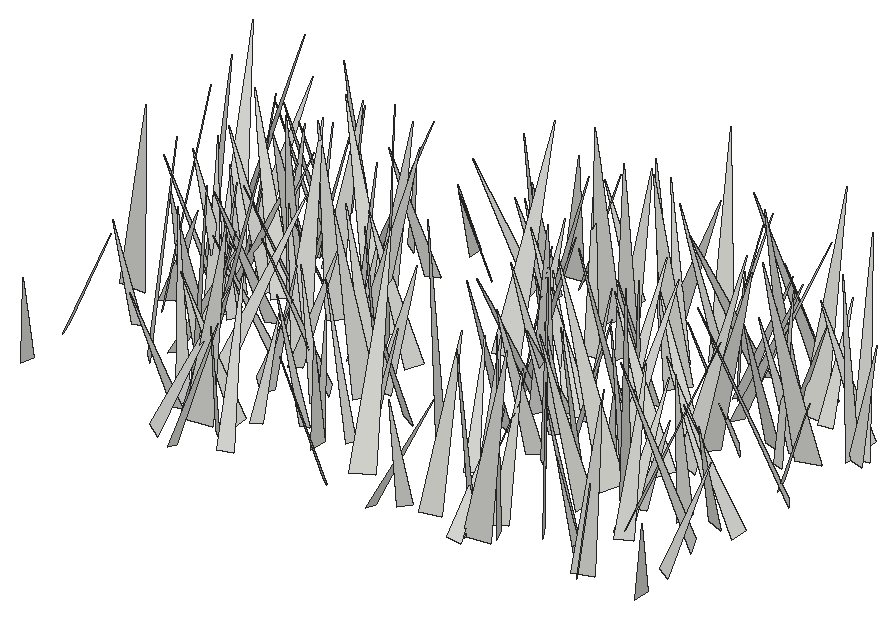
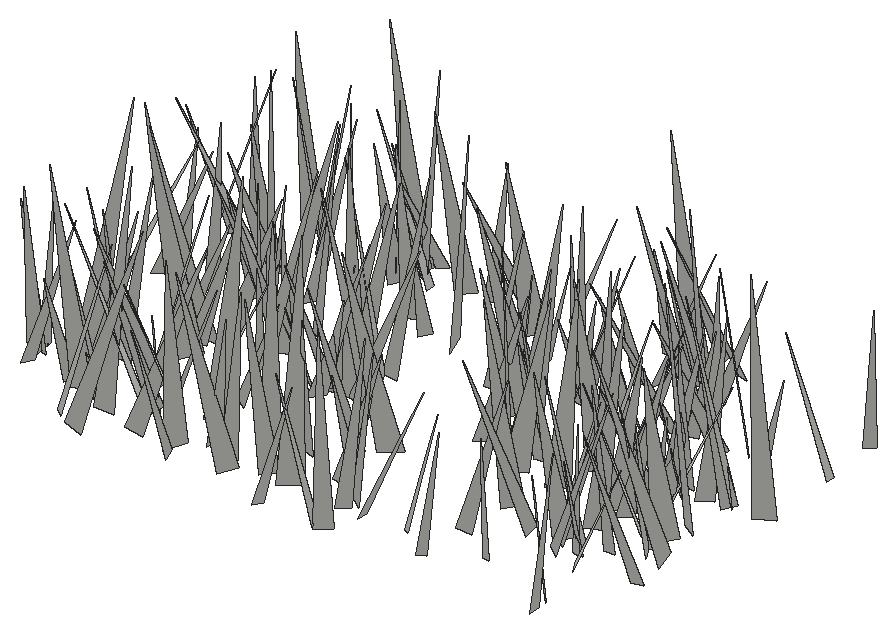
# SketchUp Ruby script. Lengths in inches.
U = 1.inch
M = Sketchup.active_model
def pt(a) = Geom::Point3d.new(a.map { |v| v * U })
def face(e, loops, mat)
  f = e.add_face(loops[0].map { |a| pt(a) })
  loops[1..].each { |l| e.add_face(l.map { |a| pt(a) }).erase! }
  f.material = f.back_material = mat if mat
  f
end
# faces: each face lists its corners as indices into pts; further lists are holes
def faces(e, pts, list, mat = nil) = list.each { |f| face(e, (f[0].is_a?(Array) ? f : [f]).map { |l| l.map { |i| pts[i] } }, mat) }
# xy, xz, yz: faces in a plane at the given z, y or x. An outline is a flat list of corners, or four numbers for a rectangle; further outlines are holes
def ring(l) = l.size == 4 ? [[l[0], l[1]], [l[2], l[1]], [l[2], l[3]], [l[0], l[3]]] : l.each_slice(2).to_a
def flat(e, list, mat, &to3) = list.each { |f| face(e, (f[0].is_a?(Array) ? f : [f]).map { |l| ring(l).map { |u, v| to3.(u, v) } }, mat) }
def xy(e, z, list, mat = nil) = flat(e, list, mat) { |x, y| [x, y, z] }
def xz(e, y, list, mat = nil) = flat(e, list, mat) { |x, z| [x, y, z] }
def yz(e, x, list, mat = nil) = flat(e, list, mat) { |y, z| [x, y, z] }
def lines(e, pts, list) = list.each { |a, b| e.add_line(pt(pts[a]), pt(pts[b])) }
# prism: a flat outline (further loops are holes) pulled along v
def prism(e, loops, v, mat = nil)
  f = face(e, loops, mat); d = Geom::Vector3d.new(v.map { |x| x * U })
  f.pushpull(f.normal.samedirection?(d) ? d.length : -d.length)
end
def box(e, o, s, mat = nil) = prism(e, [[o, [o[0] + s[0], o[1], o[2]], [o[0] + s[0], o[1] + s[1], o[2]], [o[0], o[1] + s[1], o[2]]]], [0, 0, s[2]], mat)
def at(x, y, z, deg = 0) = Geom::Transformation.translation(pt([x, y, z])) * Geom::Transformation.rotation(ORIGIN, Z_AXIS, deg.degrees)
def axes(o, x, y, z) = Geom::Transformation.new([*x, 0, *y, 0, *z, 0, *pt(o).to_a, 1])
def part(name) = M.definitions.add(name)
# library, detail: a bought-in or finely detailed component or shape, given as its bounding box
def library(name, o, s) = part(name).tap { |d| box(d.entities, o, s) }
def detail(e, o, s) = box(e.add_group.entities, o, s)
def put(e, d, t, mat = nil) = e.add_instance(d, t).tap { |i| i.material = mat if mat }
def group(e, t, mat = nil) = e.add_group.tap { |g| g.transformation = t; g.material = mat if mat }.entities
root = M.entities
c1 = part("fur_instance\#9")
p = [[0.8125,0,1.79],[0.67,-0.02,1.48],[0,-0.11,0],[0,0.11,0]]
faces(c1.entities,p,[[0,1,2,3]])
put(root,c1,axes([515.02,377.61,-21.66],[4.28943,0.41298,0.87796],[0.18379,-4.25331,1.1028],[-0.95267,1.03894,4.16576]))
put(root,c1,axes([501.53,380.35,-21.66],[3.7269,-2.05729,0.24824],[-1.97365,-3.67974,-0.86491],[-0.63149,-0.64103,4.16823]))
put(root,c1,axes([536.71,380.03,-21.66],[-1.94061,6.26278,4.61542],[7.19839,3.24975,-1.38302],[2.95087,-3.80883,6.40903]))
put(root,c1,axes([548.84,380.86,-21.66],[3.9114,-1.46291,0.01114],[-1.40736,-3.77134,-1.11157],[-0.39945,-1.03737,4.02536]))
put(root,c1,axes([516.36,380.32,-21.66],[2.79226,2.81825,2.22878],[3.51982,-2.71249,-0.9798],[-0.72174,-2.32521,3.84438]))
put(root,c1,axes([525.09,379.86,-21.66],[-2.96371,-3.18096,0.56073],[-3.21747,2.84043,-0.89238],[-0.28422,1.01488,4.25508]))
put(root,c1,axes([530.68,380.6,-21.66],[2.96444,-3.24193,0.90441],[-3.19075,-3.09049,-0.61962],[-1.07107,0.23387,4.34903]))
put(root,c1,axes([512.91,378.43,-21.66],[2.64419,5.03318,0.33977],[4.95036,-2.51506,-1.26831],[0.97076,-0.88412,5.54221]))
put(root,c1,axes([514.43,380.82,-21.66],[3.42079,-7.2545,1.9343],[-7.49487,-3.17419,1.34998],[0.44283,2.31686,7.90614]))
put(root,c1,axes([535.65,381,-21.66],[3.71105,4.69804,3.51461],[5.68502,-3.90755,-0.77947],[-1.45074,-3.29476,5.93598]))
put(root,c1,axes([529.1,379.28,-21.66],[4.45979,0.0367,0.09292],[0.01604,-4.35825,0.95137],[-0.0986,0.95079,4.35729]))
put(root,c1,axes([544.46,380.66,-21.66],[3.53738,-5.32848,1.99163],[-5.66565,-3.51029,0.67133],[-0.50966,2.039,6.36044]))
put(root,c1,axes([512.27,381.46,-21.66],[-0.63614,-4.28295,0.71253],[-4.25699,0.4736,-0.95381],[-0.85404,0.8295,4.22357]))
put(root,c1,axes([536.11,380.16,-21.66],[4.52049,-0.19473,1.20973],[-0.39564,-4.60837,0.73662],[-1.15967,0.81315,4.46432]))
put(root,c1,axes([535.64,379.1,-21.66],[-1.08496,4.24211,0.2137],[4.12597,1.10497,-0.98676],[1.00871,0.04308,4.26602]))
put(root,c1,axes([517.94,379.03,-21.66],[-0.8094,5.47668,0.09308],[5.43232,0.79056,0.72297],[-0.70181,-0.19701,5.48875]))
put(root,c1,axes([534.66,381.58,-21.66],[5.44749,2.02001,0.26599],[2.02291,-5.27178,-1.39377],[0.24298,-1.39796,5.64031]))
put(root,c1,axes([542.72,382.29,-21.66],[3.69815,0.46024,1.83595],[1.02421,-3.87534,-1.09159],[-1.5917,-1.42435,3.56322]))
put(root,c1,axes([532.54,380.76,-21.66],[-2.8521,5.31504,2.52319],[5.50682,3.39878,-0.93481],[2.07151,-1.71732,5.95905]))
put(root,c1,axes([542.52,382.71,-21.66],[-4.88015,-2.78524,1.52655],[-2.68194,5.11285,0.7548],[1.7015,0.07051,5.5681]))
put(root,c1,axes([544.2,380.46,-21.66],[4.62309,3.63215,1.82021],[3.50208,-4.96051,1.00367],[-2.05939,-0.28182,5.79293]))
put(root,c1,axes([516.47,382.34,-21.66],[-5.33847,-0.05884,0.40473],[-0.0096,5.31499,0.64603],[0.40887,-0.64342,5.29956]))
put(root,c1,axes([521.91,383.08,-21.66],[4.60045,-1.39498,0.802],[-1.20201,-4.59424,-1.0961],[-1.06973,-0.83684,4.68067]))
put(root,c1,axes([537.4,381.3125,-21.66],[-5.47988,-2.79163,2.54101],[-3.31815,5.69792,-0.89593],[1.79996,2.00489,6.08438]))
put(root,c1,axes([539.3,383.32,-21.66],[4.52719,2.71843,2.25301],[3.1828,-4.72799,-0.69084],[-1.52829,-1.79378,5.23527]))
put(root,c1,axes([513,382.04,-21.66],[-6.34859,-2.07949,3.15929],[-2.7531,6.77324,-1.07409],[2.59343,2.09974,6.59357]))
put(root,c1,axes([512.7,381.8,-21.66],[5.61181,2.09612,1.30854],[1.89864,-5.73587,1.04566],[-1.58152,0.55181,5.89854]))
put(root,c1,axes([536.69,382.27,-21.66],[3.58302,-2.92408,2.58959],[-3.63927,-3.77537,0.77237],[-1.41842,2.30013,4.5598]))
put(root,c1,axes([514.33,381.36,-21.66],[2.31766,5.02687,0.82298],[4.84651,-2.45447,1.34356],[-1.56781,-0.15629,5.3699]))
put(root,c1,axes([512.23,382.14,-21.66],[-5.96382,1.04535,0.88629],[0.82737,5.90096,-1.39268],[1.09259,1.23747,5.8924]))
put(root,c1,axes([517.27,382.95,-21.66],[-2.50227,2.59124,1.1484],[2.47228,2.74461,-0.80603],[1.38608,-0.21748,3.51087]))
put(root,c1,axes([521,384.45,-21.66],[-1.15878,-4.12917,1.68532],[-4.31214,1.48176,0.66553],[1.13832,1.40977,4.23673]))
put(root,c1,axes([548.17,383.84,-21.66],[1.81296,4.05322,0.9149],[4.0683,-1.5284,-1.29051],[0.84535,-1.3371,4.24853]))
put(root,c1,axes([519.85,384.42,-21.66],[-1.05409,-4.02831,1.60299],[-4.27873,0.70037,-1.05356],[-0.69957,1.78611,4.02845]))
put(root,c1,axes([526.15,382.11,-21.66],[-5.32969,5.59283,1.04722],[5.46672,5.43108,-1.18331],[1.57839,0.07463,7.63447]))
put(root,c1,axes([500.93,384.9,-21.66],[4.64757,1.11707,0.03174],[1.0994,-4.54603,-0.98676],[0.20042,-0.96672,4.67697]))
put(root,c1,axes([533.22,385.27,-21.66],[1.79677,-5.19077,1.98742],[-5.55817,-1.66844,0.66734],[0.02536,2.09632,5.45226]))
put(root,c1,axes([512.23,383.71,-21.66],[7.1658,2.76652,1.69463],[2.58302,-7.35112,1.0785],[-1.96302,0.42601,7.60521]))
put(root,c1,axes([510.76,386.04,-21.66],[1.65267,-3.08975,1.39314],[-3.11179,-1.99748,-0.7386],[-1.34319,0.82596,3.42525]))
put(root,c1,axes([523.22,384.66,-21.66],[-5.0928,-0.09663,0.30052],[-0.16718,4.94609,-1.24277],[0.26777,1.25023,4.93978]))
put(root,c1,axes([547.4375,387.625,-21.66],[-6.20771,-3.16783,0.82777],[-3.08728,6.25411,0.78157],[1.09042,-0.32718,6.92531]))
put(root,c1,axes([524.13,385.21,-21.66],[3.78689,-0.0231,1.24793],[-0.32688,-3.86581,0.92039],[-1.20458,0.97644,3.67342]))
put(root,c1,axes([539.24,387.36,-21.66],[-6.05597,0.77226,2.0179],[1.21073,6.18666,1.26588],[1.78953,-1.57224,5.97233]))
put(root,c1,axes([507.14,385.13,-21.66],[4.85297,5.01471,2.08252],[4.89411,-5.24941,1.23566],[-2.35199,-0.5761,6.86817]))
put(root,c1,axes([529.1,386.17,-21.66],[-7.32615,-2.19993,2.60741],[-2.57876,7.61493,-0.82074],[2.23345,1.57604,7.60517]))
put(root,c1,axes([543.68,385.6,-21.66],[3.74309,-3.05687,3.19875],[-4.02453,-4.09315,0.7978],[-1.83838,2.73658,4.76642]))
put(root,c1,axes([514.06,387.06,-21.66],[2.61371,2.45973,0.53308],[2.49517,-2.43181,-1.01309],[0.32949,-1.09634,3.44317]))
put(root,c1,axes([524.23,388.98,-21.66],[-1.58112,-4.73276,0.31075],[-4.65779,1.61119,0.83937],[0.89473,0.02406,4.91878]))
put(root,c1,axes([515.36,386.55,-21.66],[4.20313,-0.16718,1.34956],[-0.39887,-4.34286,0.70427],[-1.30006,0.79192,4.14708]))
put(root,c1,axes([518.23,388.9,-21.66],[-5.1626,-2.88411,0.4563],[-2.82641,5.16852,0.6903],[0.7333,-0.3834,5.87316]))
put(root,c1,axes([507.92,386.7,-21.66],[4.70172,-1.10111,0.26171],[-1.12934,-4.49092,1.39405],[0.07438,1.41645,4.62334]))
put(root,c1,axes([503.99,387.99,-21.66],[-0.09942,-3.58739,1.13729],[-3.70553,-0.10534,-0.65623],[-0.65715,1.13676,3.52826]))
put(root,c1,axes([518.55,387.15,-21.66],[-0.54656,4.2534,1.19948],[4.32093,0.26075,1.04426],[-0.92722,-1.29209,4.15928]))
put(root,c1,axes([531.24,386.32,-21.66],[-2.96108,3.10315,0.36366],[3.04624,2.97875,-0.6142],[0.69442,0.16515,4.24503]))
put(root,c1,axes([543.19,386.12,-21.66],[-2.46279,4.53865,0.90199],[4.34757,2.61941,-1.3098],[1.58479,-0.13272,4.99491]))
put(root,c1,axes([520.41,389.55,-21.66],[4.49335,-4.83843,2.48866],[-4.8443,-5.0271,-1.02712],[-2.47721,1.05444,6.5227]))
put(root,c1,axes([511.64,386.47,-21.66],[1.69788,6.23349,0.03172],[6.16311,-1.67374,-0.97718],[0.93461,-0.28707,6.38626]))
put(root,c1,axes([546.875,390.42,-21.66],[-0.66532,-4.77379,0.4836],[-4.67341,0.75535,1.0268],[1.0873,0.32553,4.70929]))
put(root,c1,axes([542.84,387.09,-21.66],[6.48449,2.8801,0.19854],[2.8437,-6.45643,0.78158],[-0.49773,0.63448,7.05214]))
put(root,c1,axes([536.36,390.45,-21.66],[-2.50316,-5.2047,1.47138],[-5.2002,2.76171,0.92225],[1.48721,0.89649,5.70124]))
put(root,c1,axes([532.87,390.5,-21.66],[1.51569,-5.39227,1.25729],[-5.41404,-1.71643,-0.83467],[-1.15995,0.96539,5.5387]))
put(root,c1,axes([544.9375,389.91,-21.66],[-4.81176,0.83188,2.6308],[1.27412,5.3609,0.63523],[2.44739,-1.15538,4.84165]))
put(root,c1,axes([542.14,389.1,-21.66],[2.6099,-2.39325,0.8726],[-2.54736,-2.4537,0.88934],[-0.00348,1.24593,3.42758]))
put(root,c1,axes([512.07,390.8,-21.66],[-4.07436,-2.22938,0.28557],[-2.14023,4.02883,0.91657],[0.68639,-0.67121,4.55307]))
put(root,c1,axes([539.99,390.36,-21.66],[7.38345,1.68053,2.79244],[2.22073,-7.65548,-1.26461],[-2.38543,-1.92527,7.46594]))
put(root,c1,axes([548.79,390.41,-21.66],[-4.51725,1.3418,0.80765],[1.52463,4.33149,1.33117],[0.35811,-1.51528,4.52039]))
put(root,c1,axes([529.7,391.71,-21.66],[-1.86711,-6.21996,0.83765],[-6.21183,1.95621,0.67975],[0.89595,0.60083,6.45848]))
put(root,c1,axes([505.19,391.73,-21.66],[4.3108,-3.69492,0.61953],[-3.55093,-4.33068,-1.12044],[-1.19463,-0.46051,5.56597]))
put(root,c1,axes([539.13,390.12,-21.66],[-7.00283,2.97011,1.6591],[3.21934,7.01289,1.03394],[1.10002,-1.61605,7.53606]))
put(root,c1,axes([500.92,391.32,-21.66],[1.84601,-7.44066,1.73932],[-7.59322,-1.58595,1.27441],[0.85535,1.97933,7.55956]))
put(root,c1,axes([534.02,389.87,-21.66],[3.38997,4.6985,2.258],[4.82742,-3.84601,0.75539],[-1.96736,-1.34115,5.74432]))
put(root,c1,axes([514.75,389.86,-21.66],[3.82826,-1.89723,1.31218],[-2.241,-3.66166,1.2438],[-0.54703,1.72325,4.08754]))
put(root,c1,axes([503.53,391.46,-21.66],[3.31192,-3.28223,0.0309],[-3.2384,-3.26025,0.79144],[0.53549,0.5836,4.59516]))
put(root,c1,axes([520.81,390.7,-21.66],[1.98838,-4.24744,1.75797],[-4.57109,-1.62434,1.24561],[0.4862,2.09896,4.52138]))
put(root,c1,axes([520.7,390.53,-21.66],[-4.62696,-2.40171,1.71965],[-2.7299,4.69747,-0.78458],[1.12828,1.51649,5.15378]))
put(root,c1,axes([539.83,390.57,-21.66],[-4.89428,-1.48699,1.50253],[-1.73277,4.99254,-0.70337],[1.21087,1.13406,5.0666]))
put(root,c1,axes([537.2,392.34,-21.66],[0.94706,-3.59902,0.23008],[-3.53322,-0.8783,0.80484],[0.72266,0.42244,3.63347]))
put(root,c1,axes([519.43,391.58,-21.66],[-4.54367,3.48057,1.82928],[3.81076,4.58683,0.73803],[0.96889,-1.71821,5.67579]))
put(root,c1,axes([529.92,392.11,-21.66],[6.22111,3.48137,1.76986],[3.77865,-6.20685,-1.07301],[-0.98698,-1.81924,7.04775]))
put(root,c1,axes([510.18,393.27,-21.66],[-0.32554,-5.06602,0.7464],[-4.99056,0.14633,-1.18345],[-1.14716,0.80105,4.9366]))
put(root,c1,axes([513.71,391.41,-21.66],[-0.78367,4.54033,1.31363],[4.69244,0.5877,0.76808],[-0.56674,-1.41222,4.54299]))
put(root,c1,axes([503.8,390.73,-21.66],[6.26441,4.08516,1.86388],[4.05019,-6.52197,0.68206],[-1.9387,-0.42509,7.44756]))
put(root,c1,axes([507.48,392.8,-21.66],[-4.95355,2.49117,1.9463],[2.93301,4.97148,1.10159],[1.17959,-1.90003,5.43416]))
put(root,c1,axes([507.28,391.07,-21.66],[-0.20928,5.81187,1.2771],[5.90875,0.05179,0.73257],[-0.70395,-1.2931,5.76932]))
put(root,c1,axes([532.45,393.33,-21.66],[0.82361,-5.861,1.93807],[-5.93962,-1.28507,-1.3621],[-1.68178,1.66825,5.75972]))
put(root,c1,axes([506.9,392.75,-21.66],[-4.69197,-2.31538,0.05263],[-2.28134,4.60011,-1.00642],[-0.39908,0.92541,5.13447]))
put(root,c1,axes([508.08,392.11,-21.66],[-3.93894,0.78438,0.2139],[0.7314,3.88076,-0.76228],[0.35506,0.70765,3.94328]))
put(root,c1,axes([531.32,395.36,-21.66],[3.03189,-3.59681,0.02756],[-3.43565,-2.90654,-1.37057],[-1.06494,-0.8632,4.50011]))
put(root,c1,axes([510.91,395.58,-21.66],[-3.83453,-4.44323,0.31037],[-4.29048,3.7947,1.3169],[1.19597,-0.63261,5.71941]))
put(root,c1,axes([506.93,391.99,-21.66],[2.12896,3.50938,0.78952],[3.35263,-2.26833,1.04217],[-1.30344,-0.10245,3.97015]))
put(root,c1,axes([533.06,393.24,-21.66],[0.75971,3.71481,1.88794],[3.89435,-1.31575,1.02184],[-1.48263,-1.55251,3.65142]))
put(root,c1,axes([517.31,393,-21.66],[7.2049,-3.47591,1.96261],[-3.83046,-7.15988,1.38131],[-1.1231,2.12096,7.87937]))
put(root,c1,axes([529.9,394.88,-21.66],[6.97183,-3.45055,1.53762],[-3.37643,-7.13932,-0.71191],[-1.69419,0.0288,7.74635]))
put(root,c1,axes([529.5,395.34,-21.66],[-1.20375,-5.21342,0.24756],[-5.17288,1.15789,-0.76855],[-0.69453,0.4118,5.2951]))
put(root,c1,axes([540.64,393.46,-21.66],[-4.45803,3.98436,0.74293],[4.03358,4.25341,1.39275],[-0.39655,-1.52789,5.81458]))
put(root,c1,axes([520.36,394.38,-21.66],[-4.35819,2.96505,1.59627],[3.3258,4.19926,1.28011],[0.52792,-1.97688,5.11338]))
put(root,c1,axes([512.49,392.89,-21.66],[-3.77046,5.93467,2.17976],[6.06315,4.1134,-0.71146],[1.79161,-1.43096,6.99504]))
put(root,c1,axes([536.93,394.82,-21.66],[-2.90211,-6.23156,1.67253],[-6.44447,2.71044,-1.08359],[-0.31368,1.96803,6.78825]))
put(root,c1,axes([543.29,394.49,-21.66],[-3.79672,1.89832,0.59417],[1.98792,3.66583,0.99077],[0.06937,-1.15319,4.1276]))
put(root,c1,axes([537.78,392.05,-21.66],[0.187,6.43803,0.46404],[6.40843,-0.12967,-0.78342],[0.77175,-0.48321,6.39292]))
put(root,c1,axes([516.23,394.03,-21.66],[0.00091,-3.67707,1.93886],[-4.08733,0.35251,0.67045],[0.75747,1.90654,3.61543]))
put(root,c1,axes([548.65,395.4,-21.66],[-5.4011,-4.4458,0.12135],[-4.40164,5.31613,-1.14717],[-0.63674,0.96192,6.9008]))
put(root,c1,axes([533.65,393.28,-21.66],[3.84083,1.33111,0.88578],[1.09907,-3.87194,1.0529],[-1.16125,0.73803,3.92622]))
put(root,c1,axes([510.02,395.87,-21.66],[-0.4517,-7.27096,2.0225],[-7.50286,0.65147,0.6664],[0.81515,1.96726,7.25444]))
put(root,c1,axes([516.55,393.39,-21.66],[3.29752,4.92899,1.52703],[4.76096,-3.60504,1.35547],[-1.98997,-0.45731,5.77332]))
put(root,c1,axes([503.68,395.2,-21.66],[4.80804,6.17674,2.98381],[6.78482,-4.81897,-0.95722],[-1.01068,-2.96612,7.76873]))
put(root,c1,axes([536.38,395.98,-21.66],[5.52429,1.58059,2.16664],[1.98524,-5.74559,-0.8703],[-1.80317,-1.48335,5.67966]))
put(root,c1,axes([527.5,396.15,-21.66],[7.30646,0.41261,0.41525],[0.46932,-7.23653,-1.06747],[-0.34987,-1.09065,7.23983]))
put(root,c1,axes([536.5,393.36,-21.66],[-1.23708,6.4323,0.84499],[6.38548,1.35924,-0.99849],[1.14637,-0.62994,6.47363]))
put(root,c1,axes([513.18,396.05,-21.66],[3.99451,-5.40043,2.70776],[-5.64329,-4.49426,-0.63847],[-2.15638,1.75774,6.68679]))
put(root,c1,axes([506.53,394.9375,-21.66],[0.17252,3.92598,1.26935],[3.97591,-0.49782,0.99933],[-1.10305,-1.18034,3.80058]))
put(root,c1,axes([507.77,396.24,-21.66],[-5.02237,2.51021,1.68016],[2.86774,4.98644,1.12241],[0.94877,-1.78398,5.50142]))
put(root,c1,axes([539.04,395.6,-21.66],[-4.27231,-1.94809,0.06255],[-1.87913,4.07681,-1.37844],[-0.51754,1.27912,4.48861]))
put(root,c1,axes([505.97,394.77,-21.66],[4.9565,-0.0282,0.53243],[-0.1703,-4.80111,1.33099],[-0.50525,1.34155,4.77453]))
put(root,c1,axes([547,396.68,-21.66],[4.10425,1.09153,0.3293],[1.14011,-3.92312,-1.20584],[0.00571,-1.24998,4.07214]))
put(root,c1,axes([541.01,395,-21.66],[1.96643,7.28816,1.86053],[7.47956,-1.69089,-1.28167],[0.79683,-2.11408,7.43918]))
put(root,c1,axes([511.16,397.73,-21.66],[-2.38013,-2.88459,0.25848],[-2.75196,2.35686,0.96161],[0.90246,-0.42079,3.61403]))
put(root,c1,axes([517.23,395.65,-21.66],[6.18055,4.14964,3.19418],[4.26505,-6.85588,0.65402],[-3.03836,-1.18276,7.41558]))
put(root,c1,axes([541.47,395.6875,-21.66],[-3.45745,4.3845,0.64107],[4.38114,3.2607,1.32749],[-0.66366,-1.31634,5.42361]))
put(root,c1,axes([540.75,397.31,-21.66],[6.79044,-4.4332,0.71146],[-4.48312,-6.76549,0.63187],[-0.24718,0.91888,8.0848]))
put(root,c1,axes([531.81,395.42,-21.66],[-2.66965,3.73747,0.14274],[3.69986,2.61324,0.77338],[-0.54785,-0.56423,4.52743]))
put(root,c1,axes([531.67,396.33,-21.66],[-5.56985,2.38046,0.65327],[2.45077,5.52546,0.76123],[0.29505,-0.95874,6.00918]))
put(root,c1,axes([508.24,398.6,-21.66],[4.15376,-5.21591,0.7578],[-5.12927,-4.22232,-0.94677],[-1.21268,-0.00681,6.60024]))
put(root,c1,axes([542.1875,398.65,-21.66],[-3.97091,-3.72473,0.66515],[-3.58252,4.01146,1.07602],[1.21718,-0.34456,5.33703]))
put(root,c1,axes([508.82,396.04,-21.66],[-4.49285,4.90641,0.97236],[5.00159,4.41981,0.80831],[0.04935,-1.26349,6.60342]))
put(root,c1,axes([516.4375,396.14,-21.66],[-5.45873,5.352,1.02249],[5.44819,5.38274,0.9113],[0.08123,-1.36725,7.5902]))
put(root,c1,axes([532.74,395.57,-21.66],[1.96135,3.70682,0.36248],[3.45553,-1.96392,1.38604],[-1.38968,0.34826,3.95807]))
put(root,c1,axes([503.99,398.4375,-21.66],[3.91302,0.34843,0.25725],[0.41449,-3.69091,-1.30566],[-0.12562,-1.32482,3.70519]))
put(root,c1,axes([505.79,397.22,-21.66],[4.04604,3.23344,0.3968],[3.2461,-3.94826,-0.92578],[0.27467,-0.96906,5.09593]))
put(root,c1,axes([546.5,399.97,-21.66],[1.61042,-7.88282,1.5376],[-7.97737,-1.75156,-0.62458],[-0.92985,1.37466,8.02136]))
put(root,c1,axes([543.62,400.1875,-21.66],[-0.77388,-5.77446,0.46112],[-5.72229,0.83441,0.84559],[0.90132,0.33953,5.76439]))
put(root,c1,axes([503.95,397.11,-21.66],[-5.29033,5.65073,1.03717],[5.57546,5.38985,-0.92613],[1.38587,-0.11308,7.68509]))
put(root,c1,axes([513.87,399.57,-21.66],[5.12868,-4.19399,1.94705],[-4.5125,-5.17419,0.74098],[-1.00889,1.82269,6.58361]))
put(root,c1,axes([545.2,400.51,-21.66],[0.47741,-4.86513,1.33169],[-4.92648,-0.73691,-0.92606],[-1.08291,1.20759,4.79999]))
put(root,c1,axes([534.81,399.81,-21.66],[0.7235,3.49331,2.20248],[3.65755,-1.58024,1.30491],[-1.91742,-1.69623,3.32022]))
put(root,c1,axes([505.73,400.37,-21.66],[-0.80392,-5.00028,1.94874],[-5.12712,1.2977,1.21465],[1.58527,1.66129,4.91668]))
put(root,c1,axes([503.87,398.96,-21.66],[4.42151,2.80893,1.55928],[2.73673,-4.68252,0.67492],[-1.68278,-0.23477,5.19464]))
put(root,c1,axes([545.27,398.55,-21.66],[2.35955,4.93164,1.36493],[4.86886,-2.62618,1.07189],[-1.57426,-0.73054,5.36093]))
put(root,c1,axes([502.5,399,-21.66],[7.43833,2.19546,1.23858],[2.06036,-7.51855,0.95355],[-1.45225,0.57818,7.69672]))
put(root,c1,axes([509.09,401.07,-21.66],[-2.70694,-4.99144,1.16007],[-5.08628,2.45713,-1.29614],[-0.62448,1.62351,5.52829]))
put(root,c1,axes([507.4,400.86,-21.66],[5.27684,1.71083,0.85913],[1.8324,-5.24307,-0.81398],[-0.55438,-1.04563,5.4872]))
put(root,c1,axes([523.9,398.875,-21.66],[-2.77927,7.20298,1.80131],[7.21654,3.07297,-1.15349],[1.74623,-1.2353,7.63392]))
put(root,c1,axes([507.19,401.77,-21.66],[-1.65671,-3.63214,1.3485],[-3.6613,1.94738,0.7471],[1.26719,0.87797,3.92161]))
put(root,c1,axes([534.58,402.28,-21.66],[4.88048,-6.02987,2.56967],[-6.14977,-5.32095,-0.80587],[-2.26779,1.4525,7.7155]))
put(root,c1,axes([508.95,400.75,-21.66],[3.9195,-3.82723,2.46639],[-4.43668,-3.94163,0.93419],[-1.02305,2.43088,5.39791]))
put(root,c1,axes([548.6875,401.8,-21.66],[0.22976,-4.49295,1.68417],[-4.67204,0.17468,1.10336],[1.09322,1.69077,4.36142]))
put(root,c1,axes([524.9375,400.625,-21.66],[6.05583,0.88682,1.38397],[0.67013,-6.15634,1.01257],[-1.50092,0.82941,6.03608]))
put(root,c1,axes([508.51,402.32,-21.66],[-2.89225,-3.68575,0.79235],[-3.76683,2.78458,-0.79678],[-0.15371,1.11313,4.61682]))
put(root,c1,axes([511.09,401.23,-21.66],[6.06997,0.80019,0.53139],[0.73411,-6.05703,0.73529],[-0.61948,0.66277,6.07817]))
put(root,c1,axes([539.79,401.5,-21.66],[5.54197,-0.978,0.47716],[-1.05474,-5.437,1.10644],[-0.26776,1.17482,5.51777]))
put(root,c1,axes([514.28,403.78,-21.66],[0.3349,-5.08877,0.86463],[-5.08924,-0.4702,-0.79617],[-0.86188,0.79915,5.03725]))
put(root,c1,axes([529.61,403.49,-21.66],[6.66168,-2.88093,2.18206],[-2.80757,-7.00677,-0.67958],[-2.27567,0.211,7.22605]))
put(root,c1,axes([548.28,401.99,-21.66],[-5.81537,-0.03657,1.70774],[-0.23888,6.01751,-0.6846],[1.69135,0.72416,5.77505]))
put(root,c1,axes([507.2,401.38,-21.66],[1.88548,3.67223,0.79609],[3.49899,-2.04056,1.12569],[-1.36969,-0.15771,3.97154]))
put(root,c1,axes([523.89,403.84,-21.66],[0.22156,-4.52657,1.23949],[-4.53883,-0.5223,-1.09609],[-1.19379,1.1457,4.39744]))
put(root,c1,axes([548.08,403.9,-21.66],[-5.1344,0.67452,1.09766],[0.89094,5.11676,1.02317],[0.93062,-1.17714,5.07643]))
put(root,c1,axes([506.37,402.98,-21.66],[-4.07706,-2.14403,0.24298],[-2.12817,3.90987,-1.20919],[-0.35608,1.18084,4.44491]))
put(root,c1,axes([501.99,402.3125,-21.66],[0.82135,5.31818,1.14764],[5.3338,-0.55827,-1.23031],[1.07271,-1.29616,5.2387]))
put(root,c1,axes([527.99,402.07,-21.66],[0.38602,5.6901,1.15392],[5.67114,-0.61727,1.14668],[-1.24374,-1.04858,5.58671]))
put(root,c1,axes([523.28,403.07,-21.66],[-1.54021,3.23682,1.39983],[3.28512,1.87235,-0.71486],[1.28237,-0.90889,3.51258]))
put(root,c1,axes([540.67,405.75,-21.66],[-0.69616,-7.71222,1.47846],[-7.81205,0.83092,0.65597],[0.79755,1.40715,7.71575]))
put(root,c1,axes([541.72,404.875,-21.66],[4.55769,0.07164,0.01251],[0.0727,-4.46545,-0.91231],[0.00209,-0.91239,4.46602]))
put(root,c1,axes([548.7,402.28,-21.66],[0.5538,7.06628,1.29605],[7.05626,-0.7792,1.23321],[-1.34954,-1.17443,6.97985]))
put(root,c1,axes([538.15,403.78,-21.66],[4.95013,-1.23925,0.4471],[-1.29852,-4.88303,0.8422],[-0.22245,0.9272,5.03291]))
put(root,c1,axes([537.6,406.67,-21.66],[0.04578,-6.29285,0.19538],[-6.21134,-0.07706,-1.02644],[-1.02831,0.18529,6.20874]))
put(root,c1,axes([526.07,405.875,-21.66],[5.79688,-5.3049,1.7816],[-5.31494,-6.02201,-0.63769],[-1.75142,0.71643,7.83193]))
put(root,c1,axes([538.76,404.05,-21.66],[6.16739,3.42449,0.19717],[3.4017,-6.05394,-1.25736],[0.441,-1.19388,6.94138]))
put(root,c1,axes([522.88,404.33,-21.66],[0.28684,-3.45624,1.82339],[-3.70035,-0.82791,-0.9872],[-1.25608,1.64973,3.32465]))
put(root,c1,axes([521.8,406.1,-21.66],[4.64418,-2.47093,1.08294],[-2.19439,-4.71399,-1.3452],[-1.56935,-0.72073,5.0857]))
put(root,c1,axes([538.14,403.52,-21.66],[2.54415,2.86578,1.34064],[2.68524,-2.86561,1.02977],[-1.67317,-0.2414,3.6912]))
put(root,c1,axes([517.02,405.96,-21.66],[-2.4025,-2.92839,0.44923],[-2.80853,2.4353,0.85486],[0.94311,-0.20767,3.69008]))
put(root,c1,axes([536.98,404.15,-21.66],[-5.93557,-1.05009,0.32847],[-1.08922,5.86272,-0.94003],[0.15548,0.98355,5.95399]))
put(root,c1,axes([511.06,405.67,-21.66],[-1.26744,-3.38882,1.28492],[-3.35573,1.6115,0.94004],[1.36901,0.81271,3.49382]))
put(root,c1,axes([520.22,406.2,-21.66],[-4.86082,-0.82699,0.28427],[-0.77768,4.82218,0.73078],[0.39992,-0.67448,4.87621]))
put(root,c1,axes([543.32,404.46,-21.66],[-0.77106,7.66776,2.67234],[8.04873,1.0768,-0.76736],[1.07416,-2.56446,7.66813]))
put(root,c1,axes([521.7,405.05,-21.66],[-3.13424,-4.33981,2.11732],[-4.81159,3.01955,-0.93345],[0.40688,2.2779,5.27125]))
put(root,c1,axes([544.48,404.17,-21.66],[-1.99149,3.68652,0.84504],[3.6319,2.13053,-0.73532],[1.05538,-0.37542,4.12502]))
put(root,c1,axes([542.64,407.63,-21.66],[-3.72414,-4.2026,0.59605],[-4.10843,3.76818,0.89886],[1.06672,-0.15915,5.54285]))
put(root,c1,axes([527.93,405.625,-21.66],[3.39124,-4.48702,2.29298],[-4.9912,-3.37077,0.78574],[-0.69206,2.32297,5.56924]))
put(root,c1,axes([535.83,404.05,-21.66],[3.94824,4.29759,0.4959],[4.2386,-3.97723,0.72087],[-0.86569,0.12707,5.79122]))
put(root,c1,axes([531.21,405.39,-21.66],[-0.70822,-5.57958,3.0516],[-6.3293,0.31925,-0.88519],[-0.61961,3.1164,5.55425]))
put(root,c1,axes([532.92,404.6,-21.66],[-5.60196,1.71083,0.59088],[1.59688,5.57635,-1.00614],[0.85208,0.79713,5.77032]))
put(root,c1,axes([514.48,407.7,-21.66],[3.47774,-1.50181,0.39234],[-1.2719,-3.30895,-1.39185],[-0.88975,-1.13996,3.5232]))
put(root,c1,axes([530.15,406.86,-21.66],[5.34451,-3.5502,0.35957],[-3.55754,-5.25077,1.03462],[0.27778,1.05952,6.33224]))
put(root,c1,axes([505.1,407.34,-21.66],[2.93725,2.51058,1.33666],[2.80043,-2.8887,-0.72813],[-0.49727,-1.43859,3.79478]))
put(root,c1,axes([540.76,408.66,-21.66],[-1.61608,-6.86234,1.14057],[-6.89566,1.42577,-1.19223],[-0.91789,1.37106,6.94853]))
put(root,c1,axes([521.15,408.89,-21.66],[2.32461,-5.72045,0.33614],[-5.68592,-2.25756,0.90225],[0.71192,0.64824,6.10846]))
put(root,c1,axes([534.47,406.5625,-21.66],[-6.2785,3.87073,1.88034],[3.7817,6.55006,-0.85632],[2.05354,-0.22787,7.32591]))
put(root,c1,axes([504.8,408.8,-21.66],[-4.71927,-1.33587,1.95814],[-1.09743,5.09822,0.83318],[2.10107,-0.33763,4.83341]))
put(root,c1,axes([521.92,408.7,-21.66],[4.65437,1.55789,0.49043],[1.62302,-4.57734,-0.86283],[-0.1826,-0.97553,4.83174]))
put(root,c1,axes([526.16,408.95,-21.66],[-4.20728,0.83557,0.99678],[1.00115,4.23485,0.67581],[0.83033,-0.87227,4.23588]))
put(root,c1,axes([534.18,407.56,-21.66],[4.3038,1.80689,1.01933],[1.67441,-4.41138,0.75005],[-1.22483,0.31842,4.60705]))
